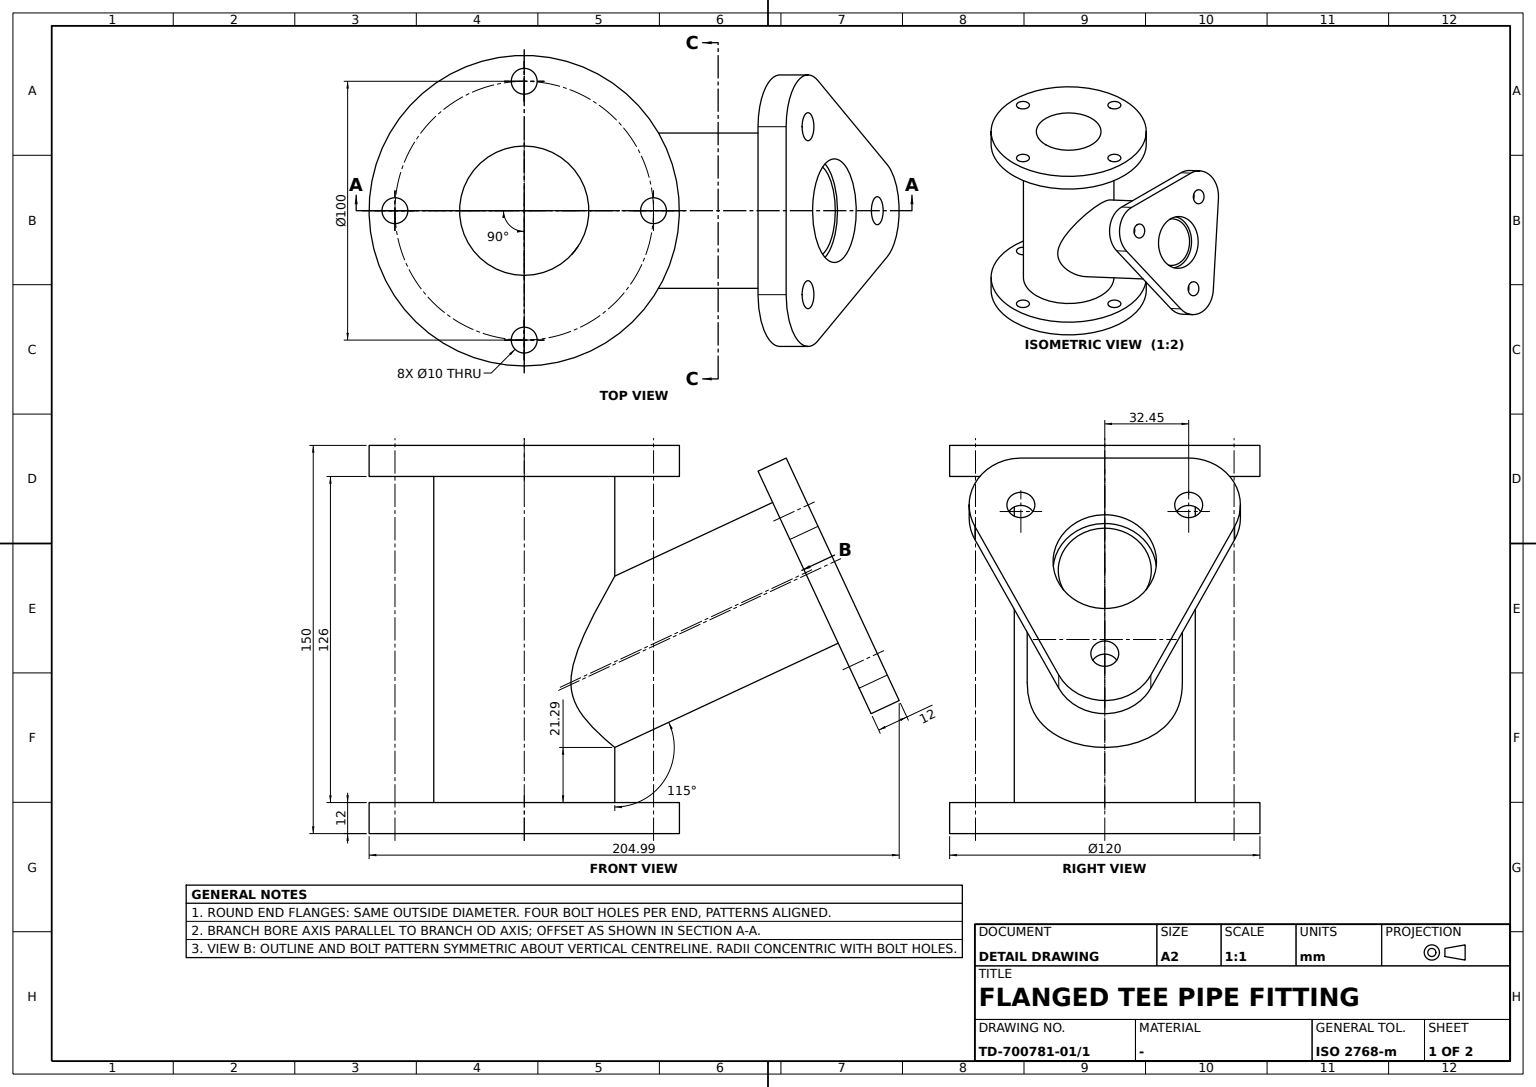
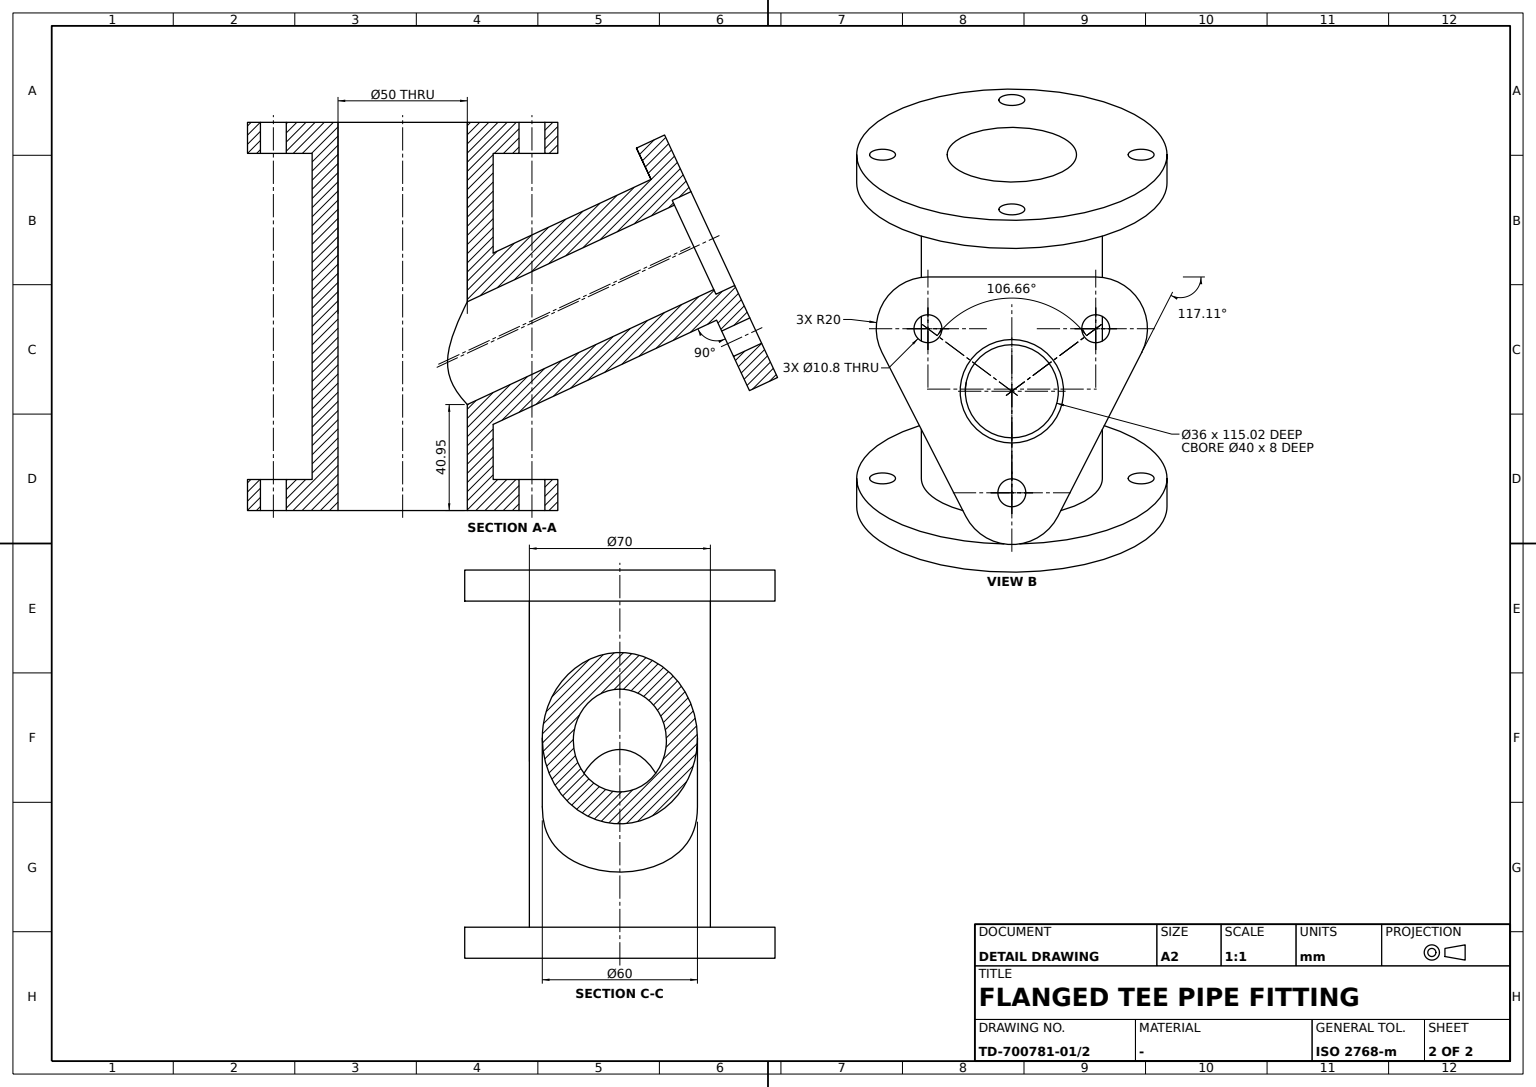
ISO-10303-21;
HEADER;
FILE_DESCRIPTION((''),'2;1');
FILE_NAME('','',(''),(''),'','','');
FILE_SCHEMA(('AUTOMOTIVE_DESIGN'));
ENDSEC;
DATA;
#1=APPLICATION_CONTEXT('');
#2=PRODUCT_CONTEXT('',#1,'mechanical');
#3=PRODUCT('','','',(#2));
#4=PRODUCT_DEFINITION_FORMATION('','',#3);
#5=PRODUCT_DEFINITION_CONTEXT('',#1,'design');
#6=PRODUCT_DEFINITION('','',#4,#5);
#7=PRODUCT_DEFINITION_SHAPE('','',#6);
#8=(LENGTH_UNIT()NAMED_UNIT(*)SI_UNIT(.MILLI.,.METRE.));
#9=(NAMED_UNIT(*)PLANE_ANGLE_UNIT()SI_UNIT($,.RADIAN.));
#10=(NAMED_UNIT(*)SI_UNIT($,.STERADIAN.)SOLID_ANGLE_UNIT());
#11=UNCERTAINTY_MEASURE_WITH_UNIT(LENGTH_MEASURE(0.005),#8,'distance_accuracy_value','');
#12=(GEOMETRIC_REPRESENTATION_CONTEXT(3)GLOBAL_UNCERTAINTY_ASSIGNED_CONTEXT((#11))GLOBAL_UNIT_ASSIGNED_CONTEXT((#8,#9,#10))REPRESENTATION_CONTEXT('',''));
#13=CARTESIAN_POINT('',(0.,96.05356,127.956666));
#14=VERTEX_POINT('',#13);
#15=CARTESIAN_POINT('',(0.,108.732108,100.767433));
#16=DIRECTION('',(0.,0.906307787,0.422618262));
#17=DIRECTION('',(0.,-0.422618262,0.906307787));
#18=AXIS2_PLACEMENT_3D('',#15,#16,#17);
#19=CIRCLE('',#18,30.);
#20=EDGE_CURVE('',#14,#14,#19,.T.);
#21=ORIENTED_EDGE('',*,*,#20,.F.);
#22=EDGE_LOOP('',(#21));
#23=FACE_BOUND('',#22,.T.);
#24=CARTESIAN_POINT('',(-30.,18.027756,58.471299));
#25=VERTEX_POINT('',#24);
#26=CARTESIAN_POINT('',(-29.576945,18.771842,51.776127));
#27=CARTESIAN_POINT('',(-30.205136,17.672315,58.491044));
#28=CARTESIAN_POINT('',(-29.602511,18.705438,65.087491));
#29=CARTESIAN_POINT('',(-28.238973,20.742889,71.320223));
#30=CARTESIAN_POINT('',(-26.266479,23.215595,77.148565));
#31=CARTESIAN_POINT('',(-23.69981,25.856281,82.6383));
#32=CARTESIAN_POINT('',(-20.415022,28.546909,87.836029));
#33=CARTESIAN_POINT('',(-16.380665,31.067847,92.490466));
#34=CARTESIAN_POINT('',(-11.396575,33.262446,96.428185));
#35=CARTESIAN_POINT('',(-5.380074,34.79033,99.120758));
#36=CARTESIAN_POINT('',(1.371541,35.193413,99.825469));
#37=CARTESIAN_POINT('',(7.930343,34.282191,98.229132));
#38=CARTESIAN_POINT('',(13.519244,32.439408,94.962114));
#39=CARTESIAN_POINT('',(18.120801,30.072217,90.671388));
#40=CARTESIAN_POINT('',(21.804604,27.487259,85.822995));
#41=CARTESIAN_POINT('',(24.800477,24.792763,80.487895));
#42=CARTESIAN_POINT('',(27.133239,22.185953,74.83953));
#43=CARTESIAN_POINT('',(28.865234,19.848552,68.858563));
#44=CARTESIAN_POINT('',(29.951548,18.11935,62.495231));
#45=CARTESIAN_POINT('',(30.136993,17.7992,55.716453));
#46=CARTESIAN_POINT('',(28.870444,19.891982,49.349793));
#47=CARTESIAN_POINT('',(26.156952,23.434784,44.256136));
#48=CARTESIAN_POINT('',(22.319437,27.155414,40.232689));
#49=CARTESIAN_POINT('',(15.848286,31.667304,36.021382));
#50=CARTESIAN_POINT('',(5.556269,35.435546,32.932286));
#51=CARTESIAN_POINT('',(-5.908464,34.991317,33.279047));
#52=CARTESIAN_POINT('',(-14.119096,32.232015,35.594425));
#53=CARTESIAN_POINT('',(-19.511632,29.260818,38.227905));
#54=CARTESIAN_POINT('',(-23.993248,25.67361,41.744934));
#55=CARTESIAN_POINT('',(-27.388876,21.951084,46.144651));
#56=B_SPLINE_CURVE_WITH_KNOTS('',3,(#26,#27,#28,#29,#30,#31,#32,#33,#34,#35,#36,#37,#38,#39,#40,#41,#42,#43,#44,#45,#46,#47,#48,#49,#50,#51,#52,#53,#54,#55,#26,#27,#28),.UNSPECIFIED.,.T.,.F.,(1,1,1,1,1,1,1,1,1,1,1,1,1,1,1,1,1,1,1,1,1,1,1,1,1,1,1,1,1,1,1,1,1,1,1,1,1),(-0.019836553,-0.013224369,-0.006612184,0.,0.006612184,0.013224369,0.019836553,0.026448737,0.033060921,0.039673106,0.04628529,0.052897474,0.059509659,0.066121843,0.072734027,0.079346211,0.085958396,0.09257058,0.099182764,0.105794948,0.112407133,0.119019317,0.125631501,0.132243686,0.13885587,0.145468054,0.158692423,0.171916791,0.178528976,0.18514116,0.191753344,0.198365528,0.204977713,0.211589897,0.218202081,0.224814266,0.23142645),.UNSPECIFIED.);
#57=EDGE_CURVE('',#25,#25,#56,.T.);
#58=ORIENTED_EDGE('',*,*,#57,.T.);
#59=EDGE_LOOP('',(#58));
#60=FACE_BOUND('',#59,.T.);
#61=CARTESIAN_POINT('',(0.,-1.337751,49.441015));
#62=DIRECTION('',(-1.,0.,0.));
#63=AXIS2_PLACEMENT_3D('',#61,#16,#62);
#64=CYLINDRICAL_SURFACE('',#63,30.);
#65=ADVANCED_FACE('',(#23,#60),#64,.T.);
#66=CARTESIAN_POINT('',(-45.,0.,0.));
#67=VERTEX_POINT('',#66);
#68=CARTESIAN_POINT('',(-50.,0.,0.));
#69=DIRECTION('',(0.,0.,1.));
#70=DIRECTION('',(1.,0.,0.));
#71=AXIS2_PLACEMENT_3D('',#68,#69,#70);
#72=CIRCLE('',#71,5.);
#73=EDGE_CURVE('',#67,#67,#72,.T.);
#74=ORIENTED_EDGE('',*,*,#73,.F.);
#75=EDGE_LOOP('',(#74));
#76=FACE_BOUND('',#75,.T.);
#77=CARTESIAN_POINT('',(-45.,0.,12.));
#78=VERTEX_POINT('',#77);
#79=CARTESIAN_POINT('',(-50.,0.,12.));
#80=AXIS2_PLACEMENT_3D('',#79,#69,#70);
#81=CIRCLE('',#80,5.);
#82=EDGE_CURVE('',#78,#78,#81,.T.);
#83=ORIENTED_EDGE('',*,*,#82,.T.);
#84=EDGE_LOOP('',(#83));
#85=FACE_BOUND('',#84,.T.);
#86=CARTESIAN_POINT('',(-50.,0.,75.));
#87=AXIS2_PLACEMENT_3D('',#86,#69,#70);
#88=CYLINDRICAL_SURFACE('',#87,5.);
#89=ADVANCED_FACE('',(#76,#85),#88,.F.);
#90=CARTESIAN_POINT('',(60.,0.,0.));
#91=VERTEX_POINT('',#90);
#92=CARTESIAN_POINT('',(0.,0.,0.));
#93=AXIS2_PLACEMENT_3D('',#92,#69,#70);
#94=CIRCLE('',#93,60.);
#95=EDGE_CURVE('',#91,#91,#94,.T.);
#96=ORIENTED_EDGE('',*,*,#95,.T.);
#97=EDGE_LOOP('',(#96));
#98=FACE_BOUND('',#97,.T.);
#99=CARTESIAN_POINT('',(60.,0.,12.));
#100=VERTEX_POINT('',#99);
#101=CARTESIAN_POINT('',(0.,0.,12.));
#102=AXIS2_PLACEMENT_3D('',#101,#69,#70);
#103=CIRCLE('',#102,60.);
#104=EDGE_CURVE('',#100,#100,#103,.T.);
#105=ORIENTED_EDGE('',*,*,#104,.F.);
#106=EDGE_LOOP('',(#105));
#107=FACE_BOUND('',#106,.T.);
#108=CARTESIAN_POINT('',(0.,0.,6.));
#109=AXIS2_PLACEMENT_3D('',#108,#69,#70);
#110=CYLINDRICAL_SURFACE('',#109,60.);
#111=ADVANCED_FACE('',(#98,#107),#110,.T.);
#112=CARTESIAN_POINT('',(32.447337,101.294515,145.11182));
#113=VERTEX_POINT('',#112);
#114=CARTESIAN_POINT('',(50.250662,113.598082,118.726737));
#115=VERTEX_POINT('',#114);
#116=CARTESIAN_POINT('',(32.447337,109.74688,126.985665));
#117=AXIS2_PLACEMENT_3D('',#116,#16,#17);
#118=CIRCLE('',#117,20.);
#119=EDGE_CURVE('',#113,#115,#118,.T.);
#120=ORIENTED_EDGE('',*,*,#119,.F.);
#121=CARTESIAN_POINT('',(32.447337,90.418822,140.040401));
#122=VERTEX_POINT('',#121);
#123=CARTESIAN_POINT('',(32.447337,95.856668,142.576111));
#124=VECTOR('',#16,1000.);
#125=LINE('',#123,#124);
#126=EDGE_CURVE('',#122,#113,#125,.T.);
#127=ORIENTED_EDGE('',*,*,#126,.F.);
#128=CARTESIAN_POINT('',(50.250662,102.722388,113.655317));
#129=VERTEX_POINT('',#128);
#130=CARTESIAN_POINT('',(32.447337,98.871187,121.914245));
#131=AXIS2_PLACEMENT_3D('',#130,#16,#17);
#132=CIRCLE('',#131,20.);
#133=EDGE_CURVE('',#122,#129,#132,.T.);
#134=ORIENTED_EDGE('',*,*,#133,.T.);
#135=CARTESIAN_POINT('',(50.250662,108.160235,116.191027));
#136=LINE('',#135,#124);
#137=EDGE_CURVE('',#129,#115,#136,.T.);
#138=ORIENTED_EDGE('',*,*,#137,.T.);
#139=EDGE_LOOP('',(#120,#127,#134,#138));
#140=FACE_BOUND('',#139,.T.);
#141=CARTESIAN_POINT('',(32.447337,104.309034,124.449955));
#142=AXIS2_PLACEMENT_3D('',#141,#16,#62);
#143=CYLINDRICAL_SURFACE('',#142,20.);
#144=ADVANCED_FACE('',(#140),#143,.T.);
#145=CARTESIAN_POINT('',(0.,104.254382,119.834753));
#146=VERTEX_POINT('',#145);
#147=CARTESIAN_POINT('',(0.,112.706747,101.708597));
#148=AXIS2_PLACEMENT_3D('',#147,#16,#17);
#149=CIRCLE('',#148,20.);
#150=EDGE_CURVE('',#146,#146,#149,.T.);
#151=ORIENTED_EDGE('',*,*,#150,.T.);
#152=EDGE_LOOP('',(#151));
#153=FACE_BOUND('',#152,.T.);
#154=CARTESIAN_POINT('',(0.,105.099619,118.022137));
#155=VERTEX_POINT('',#154);
#156=CIRCLE('',#148,18.);
#157=EDGE_CURVE('',#155,#155,#156,.T.);
#158=ORIENTED_EDGE('',*,*,#157,.F.);
#159=EDGE_LOOP('',(#158));
#160=FACE_BOUND('',#159,.T.);
#161=CARTESIAN_POINT('',(0.,131.533277,61.334974));
#162=AXIS2_PLACEMENT_3D('',#161,#16,#62);
#163=PLANE('',#162);
#164=ADVANCED_FACE('',(#153,#160),#163,.T.);
#165=CARTESIAN_POINT('',(17.803324,129.512866,56.202952));
#166=VERTEX_POINT('',#165);
#167=CARTESIAN_POINT('',(17.803324,140.38856,61.274371));
#168=VERTEX_POINT('',#167);
#169=CARTESIAN_POINT('',(17.803324,134.950713,58.738662));
#170=LINE('',#169,#124);
#171=EDGE_CURVE('',#166,#168,#170,.T.);
#172=ORIENTED_EDGE('',*,*,#171,.T.);
#173=CARTESIAN_POINT('',(15.647446,142.168582,57.4571));
#174=DIRECTION('',(0.455635937,-0.376200499,0.806764574));
#175=VECTOR('',#174,1000.);
#176=LINE('',#173,#175);
#177=EDGE_CURVE('',#168,#115,#176,.T.);
#178=ORIENTED_EDGE('',*,*,#177,.T.);
#179=ORIENTED_EDGE('',*,*,#137,.F.);
#180=CARTESIAN_POINT('',(15.647446,131.292889,52.385681));
#181=LINE('',#180,#175);
#182=EDGE_CURVE('',#166,#129,#181,.T.);
#183=ORIENTED_EDGE('',*,*,#182,.F.);
#184=EDGE_LOOP('',(#172,#178,#179,#183));
#185=FACE_BOUND('',#184,.T.);
#186=DIRECTION('',(-0.890166216,-0.192560068,0.412946398));
#187=AXIS2_PLACEMENT_3D('',#165,#186,#174);
#188=PLANE('',#187);
#189=ADVANCED_FACE('',(#185),#188,.F.);
#190=CARTESIAN_POINT('',(5.,50.,138.));
#191=VERTEX_POINT('',#190);
#192=CARTESIAN_POINT('',(0.,50.,138.));
#193=AXIS2_PLACEMENT_3D('',#192,#69,#70);
#194=CIRCLE('',#193,5.);
#195=EDGE_CURVE('',#191,#191,#194,.T.);
#196=ORIENTED_EDGE('',*,*,#195,.T.);
#197=EDGE_LOOP('',(#196));
#198=FACE_BOUND('',#197,.T.);
#199=CARTESIAN_POINT('',(55.,0.,138.));
#200=VERTEX_POINT('',#199);
#201=CARTESIAN_POINT('',(50.,0.,138.));
#202=AXIS2_PLACEMENT_3D('',#201,#69,#70);
#203=CIRCLE('',#202,5.);
#204=EDGE_CURVE('',#200,#200,#203,.T.);
#205=ORIENTED_EDGE('',*,*,#204,.T.);
#206=EDGE_LOOP('',(#205));
#207=FACE_BOUND('',#206,.T.);
#208=CARTESIAN_POINT('',(60.,0.,138.));
#209=VERTEX_POINT('',#208);
#210=CARTESIAN_POINT('',(0.,0.,138.));
#211=AXIS2_PLACEMENT_3D('',#210,#69,#70);
#212=CIRCLE('',#211,60.);
#213=EDGE_CURVE('',#209,#209,#212,.T.);
#214=ORIENTED_EDGE('',*,*,#213,.F.);
#215=EDGE_LOOP('',(#214));
#216=FACE_BOUND('',#215,.T.);
#217=CARTESIAN_POINT('',(-45.,0.,138.));
#218=VERTEX_POINT('',#217);
#219=CARTESIAN_POINT('',(-50.,0.,138.));
#220=AXIS2_PLACEMENT_3D('',#219,#69,#70);
#221=CIRCLE('',#220,5.);
#222=EDGE_CURVE('',#218,#218,#221,.T.);
#223=ORIENTED_EDGE('',*,*,#222,.T.);
#224=EDGE_LOOP('',(#223));
#225=FACE_BOUND('',#224,.T.);
#226=CARTESIAN_POINT('',(35.,0.,138.));
#227=VERTEX_POINT('',#226);
#228=CIRCLE('',#211,35.);
#229=EDGE_CURVE('',#227,#227,#228,.T.);
#230=ORIENTED_EDGE('',*,*,#229,.T.);
#231=EDGE_LOOP('',(#230));
#232=FACE_BOUND('',#231,.T.);
#233=CARTESIAN_POINT('',(5.,-50.,138.));
#234=VERTEX_POINT('',#233);
#235=CARTESIAN_POINT('',(0.,-50.,138.));
#236=AXIS2_PLACEMENT_3D('',#235,#69,#70);
#237=CIRCLE('',#236,5.);
#238=EDGE_CURVE('',#234,#234,#237,.T.);
#239=ORIENTED_EDGE('',*,*,#238,.T.);
#240=EDGE_LOOP('',(#239));
#241=FACE_BOUND('',#240,.T.);
#242=PLANE('',#211);
#243=ADVANCED_FACE('',(#198,#207,#216,#225,#232,#241),#242,.F.);
#244=CARTESIAN_POINT('',(25.,0.,150.));
#245=VERTEX_POINT('',#244);
#246=CARTESIAN_POINT('',(0.,0.,150.));
#247=AXIS2_PLACEMENT_3D('',#246,#69,#70);
#248=CIRCLE('',#247,25.);
#249=EDGE_CURVE('',#245,#245,#248,.T.);
#250=ORIENTED_EDGE('',*,*,#249,.T.);
#251=EDGE_LOOP('',(#250));
#252=FACE_BOUND('',#251,.T.);
#253=CARTESIAN_POINT('',(25.,0.,0.));
#254=VERTEX_POINT('',#253);
#255=CIRCLE('',#93,25.);
#256=EDGE_CURVE('',#254,#254,#255,.T.);
#257=ORIENTED_EDGE('',*,*,#256,.F.);
#258=EDGE_LOOP('',(#257));
#259=FACE_BOUND('',#258,.T.);
#260=CARTESIAN_POINT('',(18.,17.349352,57.242713));
#261=VERTEX_POINT('',#260);
#262=CARTESIAN_POINT('',(17.767608,17.594055,61.14837));
#263=CARTESIAN_POINT('',(18.115909,17.226857,57.236544));
#264=CARTESIAN_POINT('',(17.768756,17.594628,53.361733));
#265=CARTESIAN_POINT('',(16.195668,19.129821,48.594837));
#266=CARTESIAN_POINT('',(12.264313,22.136072,44.109265));
#267=CARTESIAN_POINT('',(5.428261,24.807402,41.140932));
#268=CARTESIAN_POINT('',(-2.491615,25.292588,40.642021));
#269=CARTESIAN_POINT('',(-9.930941,23.322762,42.73589));
#270=CARTESIAN_POINT('',(-14.579145,20.440983,46.434098));
#271=CARTESIAN_POINT('',(-16.953456,18.404667,50.613271));
#272=CARTESIAN_POINT('',(-17.928952,17.427181,54.284582));
#273=CARTESIAN_POINT('',(-18.085534,17.259343,58.256705));
#274=CARTESIAN_POINT('',(-17.436775,17.935165,63.316518));
#275=CARTESIAN_POINT('',(-15.439334,19.797962,69.248087));
#276=CARTESIAN_POINT('',(-11.482451,22.430918,75.41488));
#277=CARTESIAN_POINT('',(-6.524509,24.348722,79.368231));
#278=CARTESIAN_POINT('',(-1.500784,25.058218,80.787357));
#279=CARTESIAN_POINT('',(2.442807,24.980975,80.633869));
#280=CARTESIAN_POINT('',(6.109939,24.326971,79.320336));
#281=CARTESIAN_POINT('',(10.272082,22.956095,76.485185));
#282=CARTESIAN_POINT('',(14.136008,20.786287,71.699084));
#283=CARTESIAN_POINT('',(16.619972,18.716286,66.051227));
#284=B_SPLINE_CURVE_WITH_KNOTS('',3,(#262,#263,#264,#265,#266,#267,#268,#269,#270,#271,#272,#273,#274,#275,#276,#277,#278,#279,#280,#281,#282,#283,#262,#263,#264),.UNSPECIFIED.,.T.,.F.,(1,1,1,1,1,1,1,1,1,1,1,1,1,1,1,1,1,1,1,1,1,1,1,1,1,1,1,1,1),(-0.0154615,-0.00773075,-0.003865375,0.,0.003865375,0.00773075,0.0154615,0.02319225,0.030923,0.03865375,0.0463845,0.050249875,0.05411525,0.057980625,0.061846,0.06957675,0.0773075,0.08503825,0.088903625,0.092768999,0.096634374,0.100499749,0.108230499,0.115961249,0.119826624,0.123691999,0.127557374,0.131422749,0.139153499),.UNSPECIFIED.);
#285=EDGE_CURVE('',#261,#261,#284,.T.);
#286=ORIENTED_EDGE('',*,*,#285,.T.);
#287=EDGE_LOOP('',(#286));
#288=FACE_BOUND('',#287,.T.);
#289=CARTESIAN_POINT('',(0.,0.,75.));
#290=AXIS2_PLACEMENT_3D('',#289,#69,#70);
#291=CYLINDRICAL_SURFACE('',#290,25.);
#292=ADVANCED_FACE('',(#252,#259,#288),#291,.F.);
#293=ORIENTED_EDGE('',*,*,#285,.F.);
#294=EDGE_LOOP('',(#293));
#295=FACE_BOUND('',#294,.T.);
#296=ORIENTED_EDGE('',*,*,#157,.T.);
#297=EDGE_LOOP('',(#296));
#298=FACE_BOUND('',#297,.T.);
#299=CARTESIAN_POINT('',(0.,12.780769,55.112348));
#300=AXIS2_PLACEMENT_3D('',#299,#16,#62);
#301=CYLINDRICAL_SURFACE('',#300,18.);
#302=ADVANCED_FACE('',(#295,#298),#301,.F.);
#303=CARTESIAN_POINT('',(5.,-50.,12.));
#304=VERTEX_POINT('',#303);
#305=CARTESIAN_POINT('',(0.,-50.,12.));
#306=AXIS2_PLACEMENT_3D('',#305,#69,#70);
#307=CIRCLE('',#306,5.);
#308=EDGE_CURVE('',#304,#304,#307,.T.);
#309=ORIENTED_EDGE('',*,*,#308,.T.);
#310=EDGE_LOOP('',(#309));
#311=FACE_BOUND('',#310,.T.);
#312=CARTESIAN_POINT('',(5.,-50.,0.));
#313=VERTEX_POINT('',#312);
#314=CARTESIAN_POINT('',(0.,-50.,0.));
#315=AXIS2_PLACEMENT_3D('',#314,#69,#70);
#316=CIRCLE('',#315,5.);
#317=EDGE_CURVE('',#313,#313,#316,.T.);
#318=ORIENTED_EDGE('',*,*,#317,.F.);
#319=EDGE_LOOP('',(#318));
#320=FACE_BOUND('',#319,.T.);
#321=CARTESIAN_POINT('',(0.,-50.,75.));
#322=AXIS2_PLACEMENT_3D('',#321,#69,#70);
#323=CYLINDRICAL_SURFACE('',#322,5.);
#324=ADVANCED_FACE('',(#311,#320),#323,.F.);
#325=CARTESIAN_POINT('',(-50.250662,113.598082,118.726737));
#326=VERTEX_POINT('',#325);
#327=CARTESIAN_POINT('',(-32.447337,101.294515,145.11182));
#328=VERTEX_POINT('',#327);
#329=CARTESIAN_POINT('',(-32.447337,109.74688,126.985665));
#330=AXIS2_PLACEMENT_3D('',#329,#16,#17);
#331=CIRCLE('',#330,20.);
#332=EDGE_CURVE('',#326,#328,#331,.T.);
#333=ORIENTED_EDGE('',*,*,#332,.F.);
#334=CARTESIAN_POINT('',(-50.250662,102.722388,113.655317));
#335=VERTEX_POINT('',#334);
#336=CARTESIAN_POINT('',(-50.250662,108.160235,116.191027));
#337=LINE('',#336,#124);
#338=EDGE_CURVE('',#335,#326,#337,.T.);
#339=ORIENTED_EDGE('',*,*,#338,.F.);
#340=CARTESIAN_POINT('',(-32.447337,90.418822,140.040401));
#341=VERTEX_POINT('',#340);
#342=CARTESIAN_POINT('',(-32.447337,98.871187,121.914245));
#343=AXIS2_PLACEMENT_3D('',#342,#16,#17);
#344=CIRCLE('',#343,20.);
#345=EDGE_CURVE('',#335,#341,#344,.T.);
#346=ORIENTED_EDGE('',*,*,#345,.T.);
#347=CARTESIAN_POINT('',(-32.447337,95.856668,142.576111));
#348=LINE('',#347,#124);
#349=EDGE_CURVE('',#341,#328,#348,.T.);
#350=ORIENTED_EDGE('',*,*,#349,.T.);
#351=EDGE_LOOP('',(#333,#339,#346,#350));
#352=FACE_BOUND('',#351,.T.);
#353=CARTESIAN_POINT('',(-32.447337,104.309034,124.449955));
#354=AXIS2_PLACEMENT_3D('',#353,#16,#62);
#355=CYLINDRICAL_SURFACE('',#354,20.);
#356=ADVANCED_FACE('',(#352),#355,.T.);
#357=CARTESIAN_POINT('',(0.,90.418822,140.040401));
#358=VECTOR('',#62,1000.);
#359=LINE('',#357,#358);
#360=EDGE_CURVE('',#122,#341,#359,.T.);
#361=ORIENTED_EDGE('',*,*,#360,.F.);
#362=ORIENTED_EDGE('',*,*,#126,.T.);
#363=CARTESIAN_POINT('',(0.,101.294515,145.11182));
#364=LINE('',#363,#358);
#365=EDGE_CURVE('',#113,#328,#364,.T.);
#366=ORIENTED_EDGE('',*,*,#365,.T.);
#367=ORIENTED_EDGE('',*,*,#349,.F.);
#368=EDGE_LOOP('',(#361,#362,#366,#367));
#369=FACE_BOUND('',#368,.T.);
#370=DIRECTION('',(0.,0.422618262,-0.906307787));
#371=AXIS2_PLACEMENT_3D('',#121,#370,#62);
#372=PLANE('',#371);
#373=ADVANCED_FACE('',(#369),#372,.F.);
#374=CARTESIAN_POINT('',(0.,134.25522,74.427361));
#375=VERTEX_POINT('',#374);
#376=CARTESIAN_POINT('',(0.,136.537358,69.533299));
#377=AXIS2_PLACEMENT_3D('',#376,#16,#17);
#378=CIRCLE('',#377,5.4);
#379=EDGE_CURVE('',#375,#375,#378,.T.);
#380=ORIENTED_EDGE('',*,*,#379,.F.);
#381=EDGE_LOOP('',(#380));
#382=FACE_BOUND('',#381,.T.);
#383=CARTESIAN_POINT('',(32.447337,107.464742,131.879727));
#384=VERTEX_POINT('',#383);
#385=CIRCLE('',#117,5.4);
#386=EDGE_CURVE('',#384,#384,#385,.T.);
#387=ORIENTED_EDGE('',*,*,#386,.F.);
#388=EDGE_LOOP('',(#387));
#389=FACE_BOUND('',#388,.T.);
#390=CARTESIAN_POINT('',(0.,111.504844,123.215699));
#391=VERTEX_POINT('',#390);
#392=CARTESIAN_POINT('',(0.,119.95721,105.089543));
#393=AXIS2_PLACEMENT_3D('',#392,#16,#17);
#394=CIRCLE('',#393,20.);
#395=EDGE_CURVE('',#391,#391,#394,.T.);
#396=ORIENTED_EDGE('',*,*,#395,.F.);
#397=EDGE_LOOP('',(#396));
#398=FACE_BOUND('',#397,.T.);
#399=CARTESIAN_POINT('',(-32.447337,107.464742,131.879727));
#400=VERTEX_POINT('',#399);
#401=CIRCLE('',#330,5.4);
#402=EDGE_CURVE('',#400,#400,#401,.T.);
#403=ORIENTED_EDGE('',*,*,#402,.F.);
#404=EDGE_LOOP('',(#403));
#405=FACE_BOUND('',#404,.T.);
#406=ORIENTED_EDGE('',*,*,#119,.T.);
#407=ORIENTED_EDGE('',*,*,#177,.F.);
#408=CARTESIAN_POINT('',(-17.803324,140.38856,61.274371));
#409=VERTEX_POINT('',#408);
#410=CIRCLE('',#377,20.);
#411=EDGE_CURVE('',#168,#409,#410,.T.);
#412=ORIENTED_EDGE('',*,*,#411,.T.);
#413=CARTESIAN_POINT('',(-15.647446,142.168582,57.4571));
#414=DIRECTION('',(-0.455635937,-0.376200499,0.806764574));
#415=VECTOR('',#414,1000.);
#416=LINE('',#413,#415);
#417=EDGE_CURVE('',#409,#326,#416,.T.);
#418=ORIENTED_EDGE('',*,*,#417,.T.);
#419=ORIENTED_EDGE('',*,*,#332,.T.);
#420=ORIENTED_EDGE('',*,*,#365,.F.);
#421=EDGE_LOOP('',(#406,#407,#412,#418,#419,#420));
#422=FACE_BOUND('',#421,.T.);
#423=CARTESIAN_POINT('',(0.,138.783739,64.71592));
#424=AXIS2_PLACEMENT_3D('',#423,#16,#62);
#425=PLANE('',#424);
#426=ADVANCED_FACE('',(#382,#389,#398,#405,#422),#425,.T.);
#427=CARTESIAN_POINT('',(0.,123.379526,69.355942));
#428=VERTEX_POINT('',#427);
#429=CARTESIAN_POINT('',(0.,125.661665,64.46188));
#430=AXIS2_PLACEMENT_3D('',#429,#16,#17);
#431=CIRCLE('',#430,5.4);
#432=EDGE_CURVE('',#428,#428,#431,.T.);
#433=ORIENTED_EDGE('',*,*,#432,.F.);
#434=EDGE_LOOP('',(#433));
#435=FACE_BOUND('',#434,.T.);
#436=ORIENTED_EDGE('',*,*,#379,.T.);
#437=EDGE_LOOP('',(#436));
#438=FACE_BOUND('',#437,.T.);
#439=CARTESIAN_POINT('',(0.,131.099512,66.997589));
#440=AXIS2_PLACEMENT_3D('',#439,#16,#62);
#441=CYLINDRICAL_SURFACE('',#440,5.4);
#442=ADVANCED_FACE('',(#435,#438),#441,.F.);
#443=CARTESIAN_POINT('',(55.,0.,12.));
#444=VERTEX_POINT('',#443);
#445=CARTESIAN_POINT('',(50.,0.,12.));
#446=AXIS2_PLACEMENT_3D('',#445,#69,#70);
#447=CIRCLE('',#446,5.);
#448=EDGE_CURVE('',#444,#444,#447,.T.);
#449=ORIENTED_EDGE('',*,*,#448,.F.);
#450=EDGE_LOOP('',(#449));
#451=FACE_BOUND('',#450,.T.);
#452=ORIENTED_EDGE('',*,*,#104,.T.);
#453=EDGE_LOOP('',(#452));
#454=FACE_BOUND('',#453,.T.);
#455=ORIENTED_EDGE('',*,*,#308,.F.);
#456=EDGE_LOOP('',(#455));
#457=FACE_BOUND('',#456,.T.);
#458=CARTESIAN_POINT('',(5.,50.,12.));
#459=VERTEX_POINT('',#458);
#460=CARTESIAN_POINT('',(0.,50.,12.));
#461=AXIS2_PLACEMENT_3D('',#460,#69,#70);
#462=CIRCLE('',#461,5.);
#463=EDGE_CURVE('',#459,#459,#462,.T.);
#464=ORIENTED_EDGE('',*,*,#463,.F.);
#465=EDGE_LOOP('',(#464));
#466=FACE_BOUND('',#465,.T.);
#467=ORIENTED_EDGE('',*,*,#82,.F.);
#468=EDGE_LOOP('',(#467));
#469=FACE_BOUND('',#468,.T.);
#470=CARTESIAN_POINT('',(35.,0.,12.));
#471=VERTEX_POINT('',#470);
#472=CIRCLE('',#102,35.);
#473=EDGE_CURVE('',#471,#471,#472,.T.);
#474=ORIENTED_EDGE('',*,*,#473,.F.);
#475=EDGE_LOOP('',(#474));
#476=FACE_BOUND('',#475,.T.);
#477=PLANE('',#102);
#478=ADVANCED_FACE('',(#451,#454,#457,#466,#469,#476),#477,.T.);
#479=CARTESIAN_POINT('',(5.,50.,150.));
#480=VERTEX_POINT('',#479);
#481=CARTESIAN_POINT('',(0.,50.,150.));
#482=AXIS2_PLACEMENT_3D('',#481,#69,#70);
#483=CIRCLE('',#482,5.);
#484=EDGE_CURVE('',#480,#480,#483,.T.);
#485=ORIENTED_EDGE('',*,*,#484,.T.);
#486=EDGE_LOOP('',(#485));
#487=FACE_BOUND('',#486,.T.);
#488=ORIENTED_EDGE('',*,*,#195,.F.);
#489=EDGE_LOOP('',(#488));
#490=FACE_BOUND('',#489,.T.);
#491=CARTESIAN_POINT('',(0.,50.,75.));
#492=AXIS2_PLACEMENT_3D('',#491,#69,#70);
#493=CYLINDRICAL_SURFACE('',#492,5.);
#494=ADVANCED_FACE('',(#487,#490),#493,.F.);
#495=ORIENTED_EDGE('',*,*,#473,.T.);
#496=EDGE_LOOP('',(#495));
#497=FACE_BOUND('',#496,.T.);
#498=ORIENTED_EDGE('',*,*,#57,.F.);
#499=EDGE_LOOP('',(#498));
#500=FACE_BOUND('',#499,.T.);
#501=ORIENTED_EDGE('',*,*,#229,.F.);
#502=EDGE_LOOP('',(#501));
#503=FACE_BOUND('',#502,.T.);
#504=CYLINDRICAL_SURFACE('',#290,35.);
#505=ADVANCED_FACE('',(#497,#500,#503),#504,.T.);
#506=ORIENTED_EDGE('',*,*,#345,.F.);
#507=CARTESIAN_POINT('',(-17.803324,129.512866,56.202952));
#508=VERTEX_POINT('',#507);
#509=CARTESIAN_POINT('',(-15.647446,131.292889,52.385681));
#510=LINE('',#509,#415);
#511=EDGE_CURVE('',#508,#335,#510,.T.);
#512=ORIENTED_EDGE('',*,*,#511,.F.);
#513=CIRCLE('',#430,20.);
#514=EDGE_CURVE('',#166,#508,#513,.T.);
#515=ORIENTED_EDGE('',*,*,#514,.F.);
#516=ORIENTED_EDGE('',*,*,#182,.T.);
#517=ORIENTED_EDGE('',*,*,#133,.F.);
#518=ORIENTED_EDGE('',*,*,#360,.T.);
#519=EDGE_LOOP('',(#506,#512,#515,#516,#517,#518));
#520=FACE_BOUND('',#519,.T.);
#521=ORIENTED_EDGE('',*,*,#432,.T.);
#522=EDGE_LOOP('',(#521));
#523=FACE_BOUND('',#522,.T.);
#524=ORIENTED_EDGE('',*,*,#20,.T.);
#525=EDGE_LOOP('',(#524));
#526=FACE_BOUND('',#525,.T.);
#527=CARTESIAN_POINT('',(32.447337,96.589048,126.808307));
#528=VERTEX_POINT('',#527);
#529=CIRCLE('',#131,5.4);
#530=EDGE_CURVE('',#528,#528,#529,.T.);
#531=ORIENTED_EDGE('',*,*,#530,.T.);
#532=EDGE_LOOP('',(#531));
#533=FACE_BOUND('',#532,.T.);
#534=CARTESIAN_POINT('',(-32.447337,96.589048,126.808307));
#535=VERTEX_POINT('',#534);
#536=CIRCLE('',#343,5.4);
#537=EDGE_CURVE('',#535,#535,#536,.T.);
#538=ORIENTED_EDGE('',*,*,#537,.T.);
#539=EDGE_LOOP('',(#538));
#540=FACE_BOUND('',#539,.T.);
#541=CARTESIAN_POINT('',(0.,127.908046,59.644501));
#542=AXIS2_PLACEMENT_3D('',#541,#16,#62);
#543=PLANE('',#542);
#544=ADVANCED_FACE('',(#520,#523,#526,#533,#540),#543,.F.);
#545=CARTESIAN_POINT('',(55.,0.,0.));
#546=VERTEX_POINT('',#545);
#547=CARTESIAN_POINT('',(50.,0.,0.));
#548=AXIS2_PLACEMENT_3D('',#547,#69,#70);
#549=CIRCLE('',#548,5.);
#550=EDGE_CURVE('',#546,#546,#549,.T.);
#551=ORIENTED_EDGE('',*,*,#550,.F.);
#552=EDGE_LOOP('',(#551));
#553=FACE_BOUND('',#552,.T.);
#554=ORIENTED_EDGE('',*,*,#448,.T.);
#555=EDGE_LOOP('',(#554));
#556=FACE_BOUND('',#555,.T.);
#557=CARTESIAN_POINT('',(50.,0.,75.));
#558=AXIS2_PLACEMENT_3D('',#557,#69,#70);
#559=CYLINDRICAL_SURFACE('',#558,5.);
#560=ADVANCED_FACE('',(#553,#556),#559,.F.);
#561=ORIENTED_EDGE('',*,*,#511,.T.);
#562=ORIENTED_EDGE('',*,*,#338,.T.);
#563=ORIENTED_EDGE('',*,*,#417,.F.);
#564=CARTESIAN_POINT('',(-17.803324,134.950713,58.738662));
#565=LINE('',#564,#124);
#566=EDGE_CURVE('',#508,#409,#565,.T.);
#567=ORIENTED_EDGE('',*,*,#566,.F.);
#568=EDGE_LOOP('',(#561,#562,#563,#567));
#569=FACE_BOUND('',#568,.T.);
#570=DIRECTION('',(-0.890166216,0.192560068,-0.412946398));
#571=AXIS2_PLACEMENT_3D('',#507,#570,#414);
#572=PLANE('',#571);
#573=ADVANCED_FACE('',(#569),#572,.T.);
#574=ORIENTED_EDGE('',*,*,#530,.F.);
#575=EDGE_LOOP('',(#574));
#576=FACE_BOUND('',#575,.T.);
#577=ORIENTED_EDGE('',*,*,#386,.T.);
#578=EDGE_LOOP('',(#577));
#579=FACE_BOUND('',#578,.T.);
#580=CYLINDRICAL_SURFACE('',#142,5.4);
#581=ADVANCED_FACE('',(#576,#579),#580,.F.);
#582=ORIENTED_EDGE('',*,*,#537,.F.);
#583=EDGE_LOOP('',(#582));
#584=FACE_BOUND('',#583,.T.);
#585=ORIENTED_EDGE('',*,*,#402,.T.);
#586=EDGE_LOOP('',(#585));
#587=FACE_BOUND('',#586,.T.);
#588=CYLINDRICAL_SURFACE('',#354,5.4);
#589=ADVANCED_FACE('',(#584,#587),#588,.F.);
#590=CARTESIAN_POINT('',(5.,50.,0.));
#591=VERTEX_POINT('',#590);
#592=CARTESIAN_POINT('',(0.,50.,0.));
#593=AXIS2_PLACEMENT_3D('',#592,#69,#70);
#594=CIRCLE('',#593,5.);
#595=EDGE_CURVE('',#591,#591,#594,.T.);
#596=ORIENTED_EDGE('',*,*,#595,.F.);
#597=EDGE_LOOP('',(#596));
#598=FACE_BOUND('',#597,.T.);
#599=ORIENTED_EDGE('',*,*,#463,.T.);
#600=EDGE_LOOP('',(#599));
#601=FACE_BOUND('',#600,.T.);
#602=ADVANCED_FACE('',(#598,#601),#493,.F.);
#603=ORIENTED_EDGE('',*,*,#204,.F.);
#604=EDGE_LOOP('',(#603));
#605=FACE_BOUND('',#604,.T.);
#606=CARTESIAN_POINT('',(55.,0.,150.));
#607=VERTEX_POINT('',#606);
#608=CARTESIAN_POINT('',(50.,0.,150.));
#609=AXIS2_PLACEMENT_3D('',#608,#69,#70);
#610=CIRCLE('',#609,5.);
#611=EDGE_CURVE('',#607,#607,#610,.T.);
#612=ORIENTED_EDGE('',*,*,#611,.T.);
#613=EDGE_LOOP('',(#612));
#614=FACE_BOUND('',#613,.T.);
#615=ADVANCED_FACE('',(#605,#614),#559,.F.);
#616=ORIENTED_EDGE('',*,*,#150,.F.);
#617=EDGE_LOOP('',(#616));
#618=FACE_BOUND('',#617,.T.);
#619=ORIENTED_EDGE('',*,*,#395,.T.);
#620=EDGE_LOOP('',(#619));
#621=FACE_BOUND('',#620,.T.);
#622=CARTESIAN_POINT('',(0.,116.331978,103.39907));
#623=AXIS2_PLACEMENT_3D('',#622,#16,#62);
#624=CYLINDRICAL_SURFACE('',#623,20.);
#625=ADVANCED_FACE('',(#618,#621),#624,.F.);
#626=ORIENTED_EDGE('',*,*,#213,.T.);
#627=EDGE_LOOP('',(#626));
#628=FACE_BOUND('',#627,.T.);
#629=CARTESIAN_POINT('',(60.,0.,150.));
#630=VERTEX_POINT('',#629);
#631=CIRCLE('',#247,60.);
#632=EDGE_CURVE('',#630,#630,#631,.T.);
#633=ORIENTED_EDGE('',*,*,#632,.F.);
#634=EDGE_LOOP('',(#633));
#635=FACE_BOUND('',#634,.T.);
#636=ADVANCED_FACE('',(#628,#635),#110,.T.);
#637=CARTESIAN_POINT('',(-45.,0.,150.));
#638=VERTEX_POINT('',#637);
#639=CARTESIAN_POINT('',(-50.,0.,150.));
#640=AXIS2_PLACEMENT_3D('',#639,#69,#70);
#641=CIRCLE('',#640,5.);
#642=EDGE_CURVE('',#638,#638,#641,.T.);
#643=ORIENTED_EDGE('',*,*,#642,.T.);
#644=EDGE_LOOP('',(#643));
#645=FACE_BOUND('',#644,.T.);
#646=ORIENTED_EDGE('',*,*,#222,.F.);
#647=EDGE_LOOP('',(#646));
#648=FACE_BOUND('',#647,.T.);
#649=ADVANCED_FACE('',(#645,#648),#88,.F.);
#650=ORIENTED_EDGE('',*,*,#73,.T.);
#651=EDGE_LOOP('',(#650));
#652=FACE_BOUND('',#651,.T.);
#653=ORIENTED_EDGE('',*,*,#256,.T.);
#654=EDGE_LOOP('',(#653));
#655=FACE_BOUND('',#654,.T.);
#656=ORIENTED_EDGE('',*,*,#317,.T.);
#657=EDGE_LOOP('',(#656));
#658=FACE_BOUND('',#657,.T.);
#659=ORIENTED_EDGE('',*,*,#95,.F.);
#660=EDGE_LOOP('',(#659));
#661=FACE_BOUND('',#660,.T.);
#662=ORIENTED_EDGE('',*,*,#595,.T.);
#663=EDGE_LOOP('',(#662));
#664=FACE_BOUND('',#663,.T.);
#665=ORIENTED_EDGE('',*,*,#550,.T.);
#666=EDGE_LOOP('',(#665));
#667=FACE_BOUND('',#666,.T.);
#668=PLANE('',#93);
#669=ADVANCED_FACE('',(#652,#655,#658,#661,#664,#667),#668,.F.);
#670=ORIENTED_EDGE('',*,*,#484,.F.);
#671=EDGE_LOOP('',(#670));
#672=FACE_BOUND('',#671,.T.);
#673=ORIENTED_EDGE('',*,*,#249,.F.);
#674=EDGE_LOOP('',(#673));
#675=FACE_BOUND('',#674,.T.);
#676=ORIENTED_EDGE('',*,*,#642,.F.);
#677=EDGE_LOOP('',(#676));
#678=FACE_BOUND('',#677,.T.);
#679=ORIENTED_EDGE('',*,*,#632,.T.);
#680=EDGE_LOOP('',(#679));
#681=FACE_BOUND('',#680,.T.);
#682=ORIENTED_EDGE('',*,*,#611,.F.);
#683=EDGE_LOOP('',(#682));
#684=FACE_BOUND('',#683,.T.);
#685=CARTESIAN_POINT('',(5.,-50.,150.));
#686=VERTEX_POINT('',#685);
#687=CARTESIAN_POINT('',(0.,-50.,150.));
#688=AXIS2_PLACEMENT_3D('',#687,#69,#70);
#689=CIRCLE('',#688,5.);
#690=EDGE_CURVE('',#686,#686,#689,.T.);
#691=ORIENTED_EDGE('',*,*,#690,.F.);
#692=EDGE_LOOP('',(#691));
#693=FACE_BOUND('',#692,.T.);
#694=PLANE('',#247);
#695=ADVANCED_FACE('',(#672,#675,#678,#681,#684,#693),#694,.T.);
#696=ORIENTED_EDGE('',*,*,#690,.T.);
#697=EDGE_LOOP('',(#696));
#698=FACE_BOUND('',#697,.T.);
#699=ORIENTED_EDGE('',*,*,#238,.F.);
#700=EDGE_LOOP('',(#699));
#701=FACE_BOUND('',#700,.T.);
#702=ADVANCED_FACE('',(#698,#701),#323,.F.);
#703=ORIENTED_EDGE('',*,*,#411,.F.);
#704=ORIENTED_EDGE('',*,*,#171,.F.);
#705=ORIENTED_EDGE('',*,*,#514,.T.);
#706=ORIENTED_EDGE('',*,*,#566,.T.);
#707=EDGE_LOOP('',(#703,#704,#705,#706));
#708=FACE_BOUND('',#707,.T.);
#709=CYLINDRICAL_SURFACE('',#440,20.);
#710=ADVANCED_FACE('',(#708),#709,.T.);
#711=CLOSED_SHELL('',(#65,#89,#111,#144,#164,#189,#243,#292,#302,#324,#356,#373,#426,#442,#478,#494,#505,#544,#560,#573,#581,#589,#602,#615,#625,#636,#649,#669,#695,#702,#710));
#712=MANIFOLD_SOLID_BREP('',#711);
#713=ADVANCED_BREP_SHAPE_REPRESENTATION('',(#712),#12);
#714=SHAPE_DEFINITION_REPRESENTATION(#7,#713);
ENDSEC;
END-ISO-10303-21;
